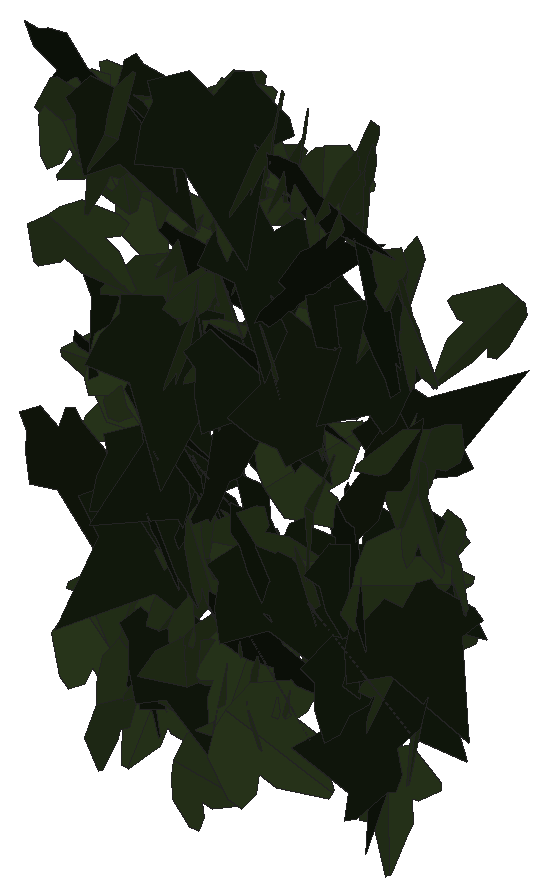
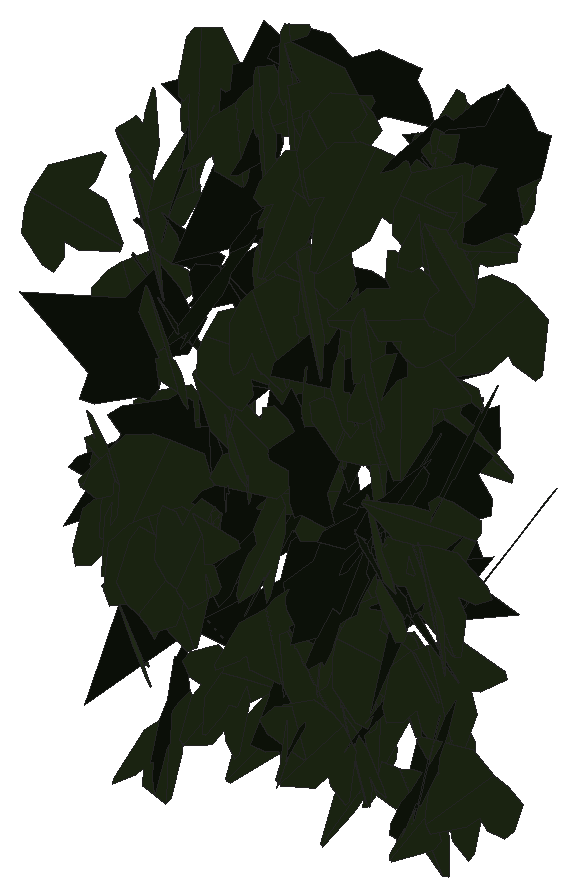
# SketchUp Ruby script. Lengths in inches.
U = 1.inch
M = Sketchup.active_model
def pt(a) = Geom::Point3d.new(a.map { |v| v * U })
def face(e, loops, mat)
  f = e.add_face(loops[0].map { |a| pt(a) })
  loops[1..].each { |l| e.add_face(l.map { |a| pt(a) }).erase! }
  f.material = f.back_material = mat if mat
  f
end
# faces: each face lists its corners as indices into pts; further lists are holes
def faces(e, pts, list, mat = nil) = list.each { |f| face(e, (f[0].is_a?(Array) ? f : [f]).map { |l| l.map { |i| pts[i] } }, mat) }
# xy, xz, yz: faces in a plane at the given z, y or x. An outline is a flat list of corners, or four numbers for a rectangle; further outlines are holes
def ring(l) = l.size == 4 ? [[l[0], l[1]], [l[2], l[1]], [l[2], l[3]], [l[0], l[3]]] : l.each_slice(2).to_a
def flat(e, list, mat, &to3) = list.each { |f| face(e, (f[0].is_a?(Array) ? f : [f]).map { |l| ring(l).map { |u, v| to3.(u, v) } }, mat) }
def xy(e, z, list, mat = nil) = flat(e, list, mat) { |x, y| [x, y, z] }
def xz(e, y, list, mat = nil) = flat(e, list, mat) { |x, z| [x, y, z] }
def yz(e, x, list, mat = nil) = flat(e, list, mat) { |y, z| [x, y, z] }
def lines(e, pts, list) = list.each { |a, b| e.add_line(pt(pts[a]), pt(pts[b])) }
# prism: a flat outline (further loops are holes) pulled along v
def prism(e, loops, v, mat = nil)
  f = face(e, loops, mat); d = Geom::Vector3d.new(v.map { |x| x * U })
  f.pushpull(f.normal.samedirection?(d) ? d.length : -d.length)
end
def box(e, o, s, mat = nil) = prism(e, [[o, [o[0] + s[0], o[1], o[2]], [o[0] + s[0], o[1] + s[1], o[2]], [o[0], o[1] + s[1], o[2]]]], [0, 0, s[2]], mat)
def at(x, y, z, deg = 0) = Geom::Transformation.translation(pt([x, y, z])) * Geom::Transformation.rotation(ORIGIN, Z_AXIS, deg.degrees)
def axes(o, x, y, z) = Geom::Transformation.new([*x, 0, *y, 0, *z, 0, *pt(o).to_a, 1])
def part(name) = M.definitions.add(name)
# library, detail: a bought-in or finely detailed component or shape, given as its bounding box
def library(name, o, s) = part(name).tap { |d| box(d.entities, o, s) }
def detail(e, o, s) = box(e.add_group.entities, o, s)
def put(e, d, t, mat = nil) = e.add_instance(d, t).tap { |i| i.material = mat if mat }
def group(e, t, mat = nil) = e.add_group.tap { |g| g.transformation = t; g.material = mat if mat }.entities
root = M.entities
M.materials.add("efeu1").color = [18, 25, 13]
M.materials.add("efeu2").color = [43, 57, 29]
c1 = part("ivyleaf_9")
p = [[1.54,2.16,1.25],[1.36,2.04,1.19],[-0.21,0.99,0.68],[-0.71,1.11,0.82],[-0.85,0.86,0.67],[-0.8,0.17,0.21],
  [-0.9,-0.01,0.1],[-0.67,-0.16,-0.02],[-0.08,-0.08,-0.05],[-0.03,-0.6,-0.4],[0.65,-0.88,-0.66],[0.83,-0.6,-0.49],
  [1.29,-0.42,-0.43],[1.8125,-0.07,-0.26],[1.21,0.44,0.15]]
faces(c1.entities,p,[[0,1,2,3,4,5,6,7,8,9,10,11,12,13,14]],"efeu1")
c2 = part("ivyleaf_10")
p = [[0,0.5,-0.03],[-0.0625,2.02,-0.43],[-0.19,2.01,-0.46],[-0.54,1.05,-0.29],[-0.52,0.625,-0.18],[-0.83,0.76,-0.28],
  [-1.16,0.64,-0.33],[-1.15,0.33,-0.24],[-0.77,-0.39,0.02],[-0.3,-0.51,0.16],[0.04,-0.48,0.23],[-0.02,2.01,-0.4375],
  [-0.06,2.01,-0.43],[0.04,-0.49,0.23],[0.67,-0.49,0.14],[1.38,0.36,-0.2],[1.375,0.51,-0.24],[0.81,0.65,-0.19],
  [0.62,0.59,-0.15],[0.6,1.09,-0.28],[0.5,1.23,-0.31]]
faces(c2.entities,p,[[0,1,2,3,4,5,6,7,8,9,10],[11,12,0,13,14,15,16,17,18,19,20]],"efeu2")
put(root,c1,axes([526.74,134.91,184.11],[-0.42318,-0.46487,-0.6064],[0.43285,0.42538,-0.62817],[0.62966,-0.60485,0.02428]))
put(root,c1,axes([525.375,135.34,176],[-0.46318,-0.51274,0.32806],[-0.22295,-0.24069,-0.69096],[0.56641,-0.51403,-0.00371]))
put(root,c2,axes([525.1875,134.34,183.26],[0.03448,-0.53503,-0.71444],[0.03351,0.71524,-0.53402],[0.89194,-0.00619,0.04768]))
put(root,c1,axes([530.41,134.64,174.35],[-0.58523,0.50797,0.40518],[-0.32983,0.23759,-0.77426],[-0.55984,-0.67099,0.03259]))
put(root,c1,axes([523.71,134.99,177.28],[0.37503,-0.69769,-0.07409],[-0.03636,0.06457,-0.7921],[0.70067,0.37678,-0.00145]))
put(root,c2,axes([527.73,134.87,180.4],[-0.40564,0.53869,-0.20779],[0.13882,-0.15551,-0.67413],[-0.56044,-0.42842,-0.01658]))
put(root,c1,axes([528.8,134.94,179.5],[-0.60122,-0.50728,0.05018],[0.09046,-0.02982,0.78246],[-0.50166,0.60257,0.08096]))
put(root,c1,axes([524.98,134.83,183.67],[0.29337,-0.65262,-0.41026],[-0.05509,0.42009,-0.70766],[0.76889,0.2791,0.10583]))
put(root,c1,axes([527.44,134.37,178.11],[-0.13811,0.5301,0.62137],[-0.20498,0.58752,-0.54679],[-0.79063,-0.24493,0.03322]))
put(root,c2,axes([527.37,134.63,176.72],[0.10466,-0.05279,0.69107],[0.50724,0.4821,-0.03999],[-0.4723,0.50607,0.11019]))
put(root,c1,axes([525.79,135.23,179.67],[-0.39072,-0.68212,-0.24032],[0.12641,0.20453,-0.78606],[0.71208,-0.41059,0.00768]))
put(root,c2,axes([524.06,134.8,182.89],[-0.24063,-0.31336,0.59718],[0.51744,0.32086,0.37686],[-0.43252,0.55819,0.11862]))
put(root,c2,axes([526.14,134.89,174.4375],[-0.18377,-0.73893,-0.18809],[0.02426,0.18771,-0.76114],[0.7621,-0.18416,-0.02112]))
put(root,c2,axes([530.14,135.29,181.34],[0.02268,-0.10955,0.76404],[0.71464,-0.28582,-0.0622],[0.29163,0.70893,0.09299]))
put(root,c2,axes([530.29,135.3,178.32],[0.19935,-0.06304,0.73639],[0.68681,-0.26595,-0.20869],[0.27302,0.71504,-0.0127]))
put(root,c1,axes([528.91,135.34,177.42],[-0.06831,-0.10657,-0.76198],[0.76567,-0.08462,-0.05681],[-0.07564,-0.76034,0.11312]))
put(root,c2,axes([528.23,135.53,177.29],[0.10553,-0.37867,-0.65909],[0.19125,-0.63077,0.39302],[-0.73567,-0.2183,0.00763]))
put(root,c2,axes([523.9,134.89,180.97],[-0.5478,-0.12381,-0.44],[0.42319,0.12217,-0.56125],[0.17274,-0.69193,-0.02037]))
put(root,c2,axes([525.03,134.97,178.82],[-0.06957,0.16608,0.73125],[-0.74985,-0.02178,-0.06639],[0.00651,-0.73423,0.16738]))
put(root,c1,axes([527.98,135.1875,182.95],[0.46574,-0.30649,0.52179],[0.45527,-0.2563,-0.55691],[0.39866,0.65075,0.02641]))
put(root,c1,axes([527.95,134.96,176.6],[-0.10301,-0.50329,-0.68042],[0.17722,0.65742,-0.5131],[0.82757,-0.20343,0.02518]))
put(root,c1,axes([528.82,134.99,175.77],[0.73771,-0.27338,-0.072],[-0.06722,0.02583,-0.78674],[0.27459,0.74077,0.00086]))
put(root,c1,axes([530.25,134.68,178.8],[-0.59328,0.2315,-0.42189],[-0.38945,0.16242,0.6368],[0.28268,0.70964,-0.00812]))
put(root,c2,axes([527.77,134.91,183.85],[0.18195,-0.75957,-0.40544],[-0.11433,0.38941,-0.78085],[0.85338,0.21412,-0.01817]))
put(root,c1,axes([523.51,135.26,183.37],[0.41819,-0.27883,0.62322],[0.50835,-0.36071,-0.50249],[0.45577,0.65816,-0.01137]))
put(root,c2,axes([526.49,134.66,172.58],[-0.07837,0.44545,0.52663],[-0.07984,0.5206,-0.45223],[-0.68512,-0.11162,-0.00754]))
put(root,c2,axes([525.1875,135.05,179.32],[0.68953,0.36327,0.25308],[0.21265,0.13908,-0.77903],[-0.38832,0.72122,0.02276]))
put(root,c1,axes([527.43,135.47,181.78],[-0.09882,-0.75434,-0.03692],[0.00481,0.0366,-0.76079],[0.75523,-0.09893,0.00001]))
put(root,c1,axes([525.58,135.18,174.42],[0.40258,-0.70404,-0.26185],[-0.11706,0.23465,-0.81089],[0.74198,0.41902,0.01414]))
put(root,c2,axes([526.1,135.11,180],[0.30195,-0.67464,-0.22854],[-0.05505,0.22538,-0.73805],[0.71017,0.30431,0.03996]))
put(root,c1,axes([527.34,134.95,177.2],[0.559,-0.33466,-0.50134],[-0.40678,0.29514,-0.65057],[0.44483,0.69044,0.0351]))
put(root,c1,axes([525.6,135.875,177.14],[-0.2297,-0.45952,0.63716],[-0.30818,-0.55792,-0.51347],[0.7226,-0.38402,-0.01644]))
put(root,c1,axes([526.99,135.18,174.88],[0.63623,-0.21354,0.49065],[0.45822,-0.17624,-0.67089],[0.27634,0.78387,-0.01718]))
put(root,c2,axes([530.44,135.35,179.28],[-0.26119,-0.70804,0.14131],[-0.05096,-0.13181,-0.75467],[0.7202,-0.26611,-0.00215]))
put(root,c2,axes([525.58,135.32,174.97],[0.65693,-0.2686,0.00963],[0.00962,-0.00194,-0.70972],[0.2686,0.657,0.00185]))
put(root,c1,axes([530.25,135.13,176.4],[-0.17582,-0.43034,-0.60026],[0.20916,0.56277,-0.46472],[0.70835,-0.27298,-0.01177]))
put(root,c2,axes([526.77,135.11,176.13],[-0.28383,0.01212,0.67893],[-0.67234,0.09805,-0.28283],[-0.09511,-0.72931,-0.02674]))
put(root,c1,axes([526.84,135.18,179.67],[0.72352,-0.22048,0.29328],[0.28814,-0.06,-0.75596],[0.22715,0.77839,0.0248]))
put(root,c2,axes([523.97,135.03,183.02],[0.26419,0.63454,0.30145],[0.06523,0.29851,-0.68552],[-0.69947,0.2675,0.04992]))
put(root,c2,axes([524.86,135.4,174.96],[-0.47405,-0.50883,0.17502],[-0.10451,-0.14174,-0.69516],[0.52784,-0.48504,0.01954]))
put(root,c2,axes([526.28,135.12,176.29],[-0.27736,0.73651,0.09498],[-0.03477,0.0884,-0.78701],[-0.7418,-0.27953,0.00138]))
put(root,c1,axes([527.15,135.21,179.9375],[0.18879,-0.65348,-0.52288],[0.01113,0.53793,-0.66827],[0.83684,0.14027,0.12685]))
put(root,c1,axes([529.7,135.5,180.52],[-0.77121,0.07208,0.10213],[-0.1019,0.00721,-0.77457],[-0.0724,-0.77791,0.00229]))
put(root,c1,axes([529.92,135.25,180.72],[0.04923,-0.60373,0.60557],[-0.06591,0.60209,0.60562],[-0.85256,-0.08141,-0.01185]))
put(root,c1,axes([525.15,135.34,178.17],[0.63291,-0.50166,-0.11268],[-0.08889,0.06926,-0.80761],[0.50642,0.63912,-0.00093]))
put(root,c2,axes([527.45,134.86,173.53],[0.21371,0.57914,0.6447],[0.19946,0.61332,-0.61706],[-0.84336,0.2918,0.01743]))
put(root,c2,axes([529.69,135.66,175.01],[0.13399,-0.61287,0.3068],[0.10096,-0.29155,-0.62649],[0.67789,0.16455,0.03266]))
put(root,c1,axes([528.4,134.66,181.63],[0.24179,0.56096,0.59216],[0.22498,0.54781,-0.61081],[-0.78404,0.33019,0.00734]))
put(root,c2,axes([526.63,135.25,183.63],[0.37721,0.16897,0.68103],[0.63871,0.23746,-0.41268],[-0.29052,0.74142,-0.02303]))
put(root,c2,axes([526.83,135.44,174.19],[0.70695,-0.05943,-0.10901],[-0.10756,0.0216,-0.70933],[0.06201,0.71498,0.01236]))
put(root,c2,axes([529.88,134.86,176.94],[-0.13388,-0.21487,-0.80094],[0.47156,0.64764,-0.25257],[0.68214,-0.48988,0.0174]))
put(root,c1,axes([524.17,135.36,178.42],[0.70748,-0.2876,0.34109],[0.31517,-0.13042,-0.7637],[0.31579,0.77451,-0.00194]))
put(root,c2,axes([527.84,135.4,176.35],[-0.57454,0.52626,-0.26037],[0.19477,-0.17284,-0.77912],[-0.55391,-0.60665,-0.00389]))
put(root,c1,axes([525.34,135.56,177.27],[-0.26803,-0.61427,-0.44928],[0.23355,0.38695,-0.66838],[0.72431,-0.35208,0.04926]))
put(root,c2,axes([525.7,136.02,175.28],[0.02413,-0.51784,0.66794],[0.06413,-0.66516,-0.518],[0.84272,0.06545,0.02029]))
put(root,c2,axes([525.39,135.23,182.49],[0.3135,-0.11368,-0.65168],[-0.51575,0.4096,-0.31956],[0.41426,0.59598,0.09532]))
put(root,c2,axes([525.74,135.48,178.27],[0.28436,-0.74754,-0.14267],[-0.03315,0.13999,-0.79959],[0.76031,0.28569,0.01849]))
put(root,c2,axes([524.68,135.82,182.82],[-0.20362,-0.13137,0.67808],[-0.47446,-0.48713,-0.23685],[0.50193,-0.51376,0.05119]))
put(root,c2,axes([524.47,135.43,182.34],[-0.39888,-0.57839,-0.13095],[0.05905,0.11829,-0.70236],[0.59008,-0.40282,-0.01823]))
put(root,c1,axes([525.25,135.2,176.55],[0.51904,-0.11952,-0.56893],[-0.53129,0.2121,-0.52926],[0.23601,0.74034,0.05978]))
put(root,c2,axes([526.04,135.74,173.72],[0.61619,-0.39934,0.27306],[0.22526,-0.15449,-0.73424],[0.42813,0.65604,-0.00668]))
put(root,c1,axes([526.8,135.9,174.19],[0.53959,-0.10676,-0.6499],[0.63451,-0.14097,0.54997],[-0.17656,-0.83286,-0.00978]))
put(root,c2,axes([529.29,136.05,181.3],[0.05926,-0.18184,0.72332],[0.36201,-0.62738,-0.18738],[0.65208,0.36482,0.03829]))
put(root,c2,axes([524.68,134.93,173.08],[-0.00232,-0.30338,-0.83146],[0.15905,0.81778,-0.29883],[0.87067,-0.1502,0.05238]))
put(root,c1,axes([524.58,136.13,173.31],[0.02167,-0.38397,0.73859],[0.13444,-0.72753,-0.38217],[0.82151,0.12919,0.04306]))
put(root,c2,axes([526.97,135.67,179.25],[0.30145,-0.00002,-0.75208],[-0.75014,-0.05807,-0.30067],[-0.05389,0.80816,-0.02162]))
put(root,c1,axes([524.6,136.11,173.16],[-0.00278,-0.18732,0.78527],[0.02239,-0.78499,-0.18718],[0.80699,0.02114,0.0079]))
put(root,c1,axes([529.46,135.21,177.21],[0.04283,-0.2263,-0.77949],[0.16775,0.76619,-0.21322],[0.79416,-0.14963,0.08708]))
put(root,c2,axes([525.04,135.63,173.09],[0.70161,-0.08805,-0.14276],[-0.13982,0.03209,-0.70697],[0.09264,0.71527,0.01415]))
put(root,c2,axes([527.15,134.95,182.27],[-0.04317,0.05821,0.81046],[-0.20593,0.78432,-0.06731],[-0.78602,-0.20868,-0.02688]))
put(root,c2,axes([527.64,135.7,180.69],[0.2356,-0.73119,-0.00605],[-0.0016,0.00584,-0.76821],[0.73122,0.2356,0.00027]))
put(root,c2,axes([527.87,135.5,183.46],[0.19698,-0.64033,-0.29423],[-0.06992,0.28624,-0.66975],[0.70121,0.20842,0.01587]))
put(root,c2,axes([529.01,135.47,183.66],[0.05908,-0.70184,-0.30774],[-0.01737,0.30735,-0.70428],[0.76615,0.06109,0.00777]))
put(root,c2,axes([528.2,135.37,179.39],[-0.43618,0.60527,0.23711],[-0.14594,0.18707,-0.74601],[-0.63346,-0.45986,0.00861]))
put(root,c2,axes([529.04,135.5625,183.22],[0.16062,-0.689,-0.23034],[0.00674,0.2373,-0.70514],[0.72645,0.15014,0.05747]))
put(root,c1,axes([523.77,136.3,178.95],[0.01681,-0.46123,0.64664],[0.03298,-0.64582,-0.4615],[0.79359,0.03661,0.00548]))
put(root,c2,axes([528.21,135.76,183.07],[0.10015,0.68433,-0.17615],[-0.05648,-0.16959,-0.69095],[-0.70438,0.11089,0.03036]))
put(root,c2,axes([525.75,136.06,179.92],[0.05253,-0.60983,0.38108],[0.03224,-0.37972,-0.61209],[0.71838,0.06164,-0.0004]))
put(root,c2,axes([526.42,135.79,179.5],[-0.02169,-0.71602,-0.0118],[0.00744,0.01158,-0.71631],[0.71607,-0.02181,0.00709]))
put(root,c2,axes([525.89,135.77,179.47],[-0.29807,0.62076,-0.2373],[0.1041,-0.21325,-0.68862],[-0.65637,-0.31572,-0.00145]))
put(root,c2,axes([526.4,135.96,174.74],[-0.44016,0.34897,0.46675],[0.37003,-0.28454,0.56169],[0.45024,0.57501,-0.00532]))
put(root,c1,axes([525.61,135.85,176.88],[-0.71764,0.32819,-0.21715],[0.19868,-0.08768,-0.78912],[-0.33969,-0.74463,-0.00279]))
put(root,c2,axes([527.53,135.69,177.625],[0.53952,-0.02131,-0.63672],[0.63533,-0.04373,0.5398],[-0.04713,-0.83342,-0.01204]))
put(root,c2,axes([530.21,135.85,175.86],[-0.38534,-0.60102,0.0939],[-0.04871,-0.08031,-0.71394],[0.60636,-0.3884,0.00232]))
put(root,c2,axes([523.73,135.7,173.63],[0.499,0.19908,0.54455],[0.50543,0.20268,-0.53724],[-0.2841,0.71025,0.00067]))
put(root,c2,axes([526.3,136.13,183.59],[0.03105,-0.66909,0.33814],[0.11154,-0.33053,-0.66429],[0.74133,0.07776,0.08579]))
put(root,c2,axes([527.91,136.24,179.59],[-0.22063,-0.17164,0.69378],[-0.33316,-0.61767,-0.25876],[0.63229,-0.38535,0.10574]))
put(root,c2,axes([526.35,135.94,180.8125],[-0.20469,-0.18173,0.70751],[0.7293,-0.0093,0.20861],[-0.0413,0.73646,0.17722]))
put(root,c2,axes([526.53,135.77,179.5625],[-0.57221,0.42577,-0.3097],[-0.24746,0.18623,0.71324],[0.46472,0.62343,-0.00154]))
put(root,c2,axes([526.35,135.83,173.78],[-0.3391,-0.65241,0.26453],[0.1171,0.23725,0.73526],[-0.69419,0.35871,-0.00519]))
put(root,c2,axes([527.26,135.36,173.73],[-0.17151,0.19933,0.78904],[-0.49314,0.61602,-0.26281],[-0.64741,-0.52204,-0.00884]))
put(root,c2,axes([529.7,136.31,174.62],[0.45257,-0.45606,0.49666],[0.34963,-0.35274,-0.6425],[0.57655,0.57189,-0.00023]))
put(root,c1,axes([529.125,135.66,175.2],[0.02554,-0.42179,-0.76247],[-0.02718,0.76204,-0.42246],[0.87093,0.03615,0.00917]))
put(root,c1,axes([525.89,136.39,176.18],[0.66776,-0.3612,-0.15555],[0.13882,-0.0703,0.75917],[-0.36795,-0.68202,0.00413]))
put(root,c2,axes([529.3,135.93,178.55],[0.69896,-0.30376,-0.00274],[0.00825,0.01211,0.76198],[-0.30366,-0.69886,0.01439]))
put(root,c1,axes([528.86,136.45,173.53],[0.01382,0.00313,-0.8044],[0.68758,-0.41761,0.01018],[-0.4175,-0.68765,-0.00985]))
put(root,c2,axes([524.03,135.84,181.7],[0.2778,-0.63305,0.29001],[-0.10842,0.26911,0.69127],[-0.68783,-0.2981,0.00817]))
put(root,c2,axes([525,136.13,176.29],[0.53974,-0.62544,-0.17542],[0.11129,-0.13566,0.82612],[-0.63997,-0.55108,-0.00428]))
put(root,c2,axes([526.93,135.76,182.47],[-0.22409,-0.56013,-0.4322],[0.14244,0.40836,-0.60308],[0.693,-0.26506,-0.0158]))
put(root,c2,axes([528.53,136.55,175.88],[-0.14152,-0.35235,-0.59672],[-0.03997,-0.60387,0.36605],[-0.69183,0.10697,0.10092]))
put(root,c1,axes([528.02,136.16,180.68],[0.4853,-0.62679,-0.07712],[-0.04666,0.0614,-0.79271],[0.62979,0.48754,0.00069]))
put(root,c1,axes([525.27,135.98,180.51],[0.6666,-0.16878,0.32157],[0.30446,-0.1067,-0.68714],[0.19798,0.73237,-0.026]))
put(root,c2,axes([529.1875,136.11,172.81],[0.05044,0.73022,-0.15348],[-0.02038,-0.15243,-0.73189],[-0.7459,0.05355,0.00962]))
put(root,c1,axes([527.07,135.88,177.76],[0.11509,-0.18919,0.79245],[-0.46025,0.64529,0.2209],[-0.67227,-0.47416,-0.01557]))
put(root,c2,axes([524.38,136.17,177.23],[0.78897,0.03802,-0.10984],[-0.10968,-0.006,-0.78989],[-0.03849,0.79656,-0.00071]))
put(root,c2,axes([529.99,136.45,176.84],[-0.13612,0.09116,-0.71728],[0.44004,-0.5687,-0.15579],[-0.57373,-0.45782,0.0507]))
put(root,c2,axes([529.53,135.88,176.87],[-0.53274,-0.54992,-0.3576],[0.2322,0.27276,-0.76536],[0.61349,-0.58077,-0.02085]))
put(root,c2,axes([528.08,136.11,173.89],[-0.56002,0.27968,-0.34624],[0.31576,-0.14253,-0.62586],[-0.31368,-0.6428,-0.01187]))
put(root,c2,axes([524.86,136.11,180.07],[-0.44213,-0.57436,-0.02969],[0.01936,0.02257,-0.72482],[0.5748,-0.44255,0.00157]))
put(root,c2,axes([525.3,136.1875,179.05],[-0.68904,-0.3434,0.20197],[0.18138,0.08886,0.76987],[-0.35471,0.71251,0.00133]))
put(root,c2,axes([527.67,136.53,174.45],[0.08962,0.41437,-0.55894],[-0.09969,-0.5501,-0.4238],[-0.6886,0.13357,-0.01139]))
put(root,c2,axes([525.65,135.99,183.125],[-0.52718,-0.47,-0.32575],[0.24085,0.21935,-0.70626],[0.51865,-0.57958,-0.00313]))
put(root,c1,axes([525.54,136.68,176.14],[0.17099,-0.49134,0.58275],[0.17584,-0.5557,-0.52013],[0.74168,0.24502,-0.01103]))
put(root,c2,axes([524.51,135.97,181.16],[0.1445,0.07148,0.74661],[0.65116,0.36535,-0.161],[-0.37219,0.66695,0.00818]))
put(root,c2,axes([530.83,136.68,181.11],[-0.05663,-0.4593,0.55048],[-0.08529,-0.54395,-0.46263],[0.71184,-0.10171,-0.01164]))
put(root,c2,axes([526.11,136.27,173.82],[-0.5319,0.07988,-0.40814],[0.38621,-0.15094,-0.53286],[-0.15428,-0.65324,0.07322]))
put(root,c1,axes([529.64,135.9,178.7],[0.01944,-0.0347,0.76344],[0.72247,0.24983,-0.00704],[-0.24917,0.72167,0.03915]))
put(root,c2,axes([524.01,136.01,177.76],[0.29625,-0.02612,-0.6077],[0.5709,0.24521,0.26777],[0.20991,-0.63003,0.12941]))
put(root,c2,axes([527.13,136.37,175.43],[0.18256,0.62411,-0.20624],[-0.06823,-0.1949,-0.65018],[-0.65376,0.19462,0.01027]))
put(root,c2,axes([529.49,136.29,181.49],[0.41713,-0.58263,-0.14501],[-0.08741,0.11576,-0.71655],[0.59401,0.42618,-0.00361]))
put(root,c2,axes([526.52,136.22,181.22],[0.27852,-0.62264,-0.23066],[-0.10983,0.20348,-0.6819],[0.65484,0.29896,-0.01627]))
put(root,c2,axes([527.1,136.54,180.58],[-0.14298,-0.65516,0.24738],[0.09313,-0.26803,-0.65602],[0.69409,-0.099,0.13898]))
put(root,c2,axes([524.29,136.24,177.25],[0.37369,-0.61341,-0.26092],[-0.13423,0.22375,-0.71827],[0.65294,0.39707,0.00167]))
put(root,c2,axes([525.26,136.32,180.79],[0.09196,-0.68411,-0.08529],[-0.02225,0.08306,-0.69018],[0.68905,0.09398,-0.0109]))
put(root,c2,axes([529.07,136.47,176.03],[-0.54464,-0.5294,0.27577],[-0.17998,-0.2103,-0.75917],[0.56915,-0.57311,0.02383]))
put(root,c2,axes([528.89,136.8,175.47],[-0.19434,-0.36266,-0.60894],[-0.29697,-0.53165,0.4114],[-0.64353,0.35485,-0.00596]))
